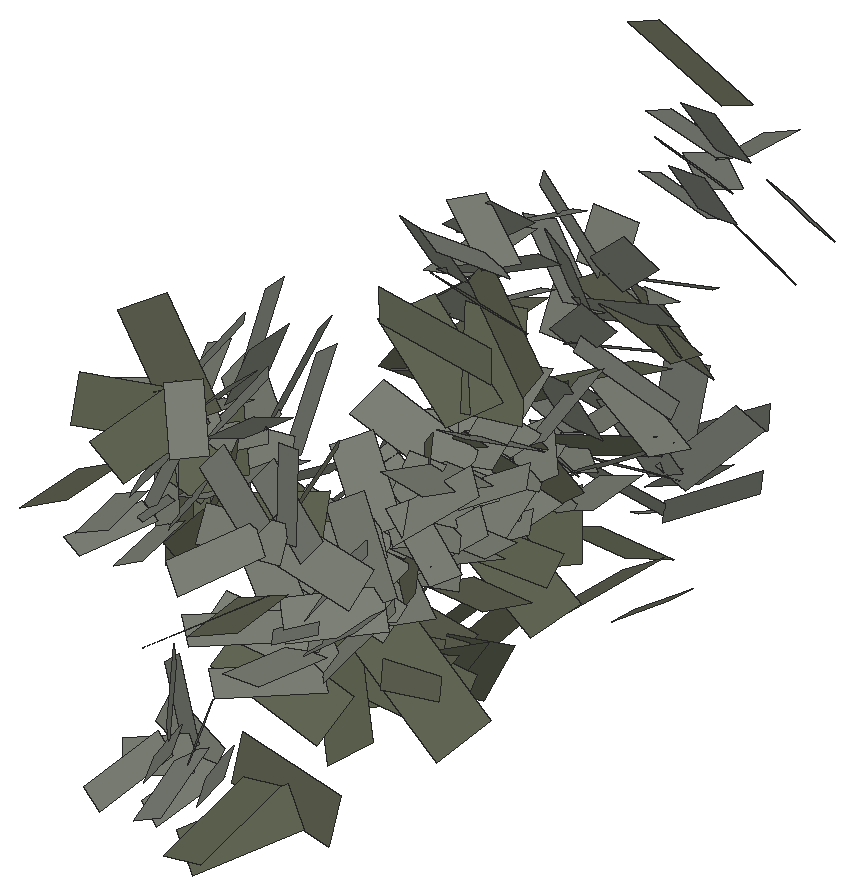
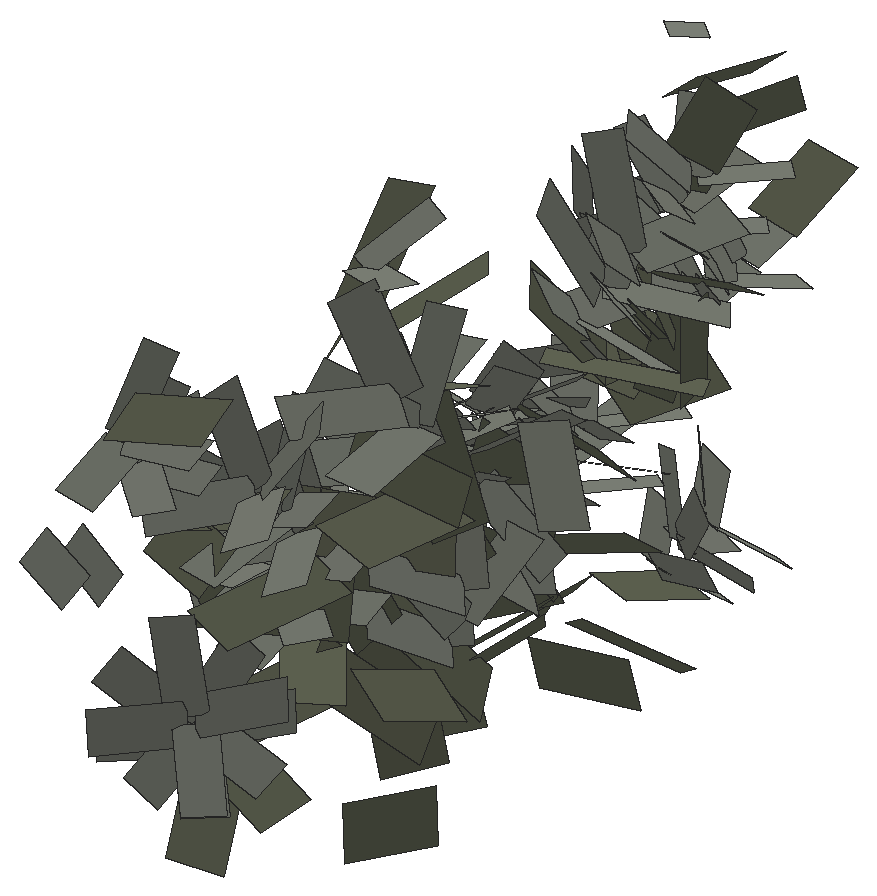
# SketchUp Ruby script. Lengths in inches.
U = 1.inch
M = Sketchup.active_model
def pt(a) = Geom::Point3d.new(a.map { |v| v * U })
def face(e, loops, mat)
  f = e.add_face(loops[0].map { |a| pt(a) })
  loops[1..].each { |l| e.add_face(l.map { |a| pt(a) }).erase! }
  f.material = f.back_material = mat if mat
  f
end
# faces: each face lists its corners as indices into pts; further lists are holes
def faces(e, pts, list, mat = nil) = list.each { |f| face(e, (f[0].is_a?(Array) ? f : [f]).map { |l| l.map { |i| pts[i] } }, mat) }
# xy, xz, yz: faces in a plane at the given z, y or x. An outline is a flat list of corners, or four numbers for a rectangle; further outlines are holes
def ring(l) = l.size == 4 ? [[l[0], l[1]], [l[2], l[1]], [l[2], l[3]], [l[0], l[3]]] : l.each_slice(2).to_a
def flat(e, list, mat, &to3) = list.each { |f| face(e, (f[0].is_a?(Array) ? f : [f]).map { |l| ring(l).map { |u, v| to3.(u, v) } }, mat) }
def xy(e, z, list, mat = nil) = flat(e, list, mat) { |x, y| [x, y, z] }
def xz(e, y, list, mat = nil) = flat(e, list, mat) { |x, z| [x, y, z] }
def yz(e, x, list, mat = nil) = flat(e, list, mat) { |y, z| [x, y, z] }
def lines(e, pts, list) = list.each { |a, b| e.add_line(pt(pts[a]), pt(pts[b])) }
# prism: a flat outline (further loops are holes) pulled along v
def prism(e, loops, v, mat = nil)
  f = face(e, loops, mat); d = Geom::Vector3d.new(v.map { |x| x * U })
  f.pushpull(f.normal.samedirection?(d) ? d.length : -d.length)
end
def box(e, o, s, mat = nil) = prism(e, [[o, [o[0] + s[0], o[1], o[2]], [o[0] + s[0], o[1] + s[1], o[2]], [o[0], o[1] + s[1], o[2]]]], [0, 0, s[2]], mat)
def at(x, y, z, deg = 0) = Geom::Transformation.translation(pt([x, y, z])) * Geom::Transformation.rotation(ORIGIN, Z_AXIS, deg.degrees)
def axes(o, x, y, z) = Geom::Transformation.new([*x, 0, *y, 0, *z, 0, *pt(o).to_a, 1])
def part(name) = M.definitions.add(name)
# library, detail: a bought-in or finely detailed component or shape, given as its bounding box
def library(name, o, s) = part(name).tap { |d| box(d.entities, o, s) }
def detail(e, o, s) = box(e.add_group.entities, o, s)
def put(e, d, t, mat = nil) = e.add_instance(d, t).tap { |i| i.material = mat if mat }
def group(e, t, mat = nil) = e.add_group.tap { |g| g.transformation = t; g.material = mat if mat }.entities
root = M.entities
M.materials.add("viburnumblaasdfas0df1w06d").color = [98, 102, 84]
M.materials.add("viburnumbladsadfasdfad0w122").color = [125, 129, 119]
c1 = part("Component\#315")
p = [[0.25,0,0],[2.05,0.01,0.35],[1.81,4.2,1.66],[0,4.19,1.3125]]
faces(c1.entities,p,[[0,1,2,3]],"viburnumbladsadfasdfad0w122")
c2 = part("viburnumblad2")
put(c2.entities,c1,axes([-19.23,-4.49,-32.18],[83.35428,0,0],[0,79.38502,0],[0,0,83.35428]))
c3 = part("Component\#314")
p = [[0.14,0,0],[2.58,0.05,0.25],[2.44,5.11,2.64],[0,5.05,2.39]]
faces(c3.entities,p,[[0,1,2,3]],"viburnumblaasdfas0df1w06d")
c4 = part("viburnumblad1\#2")
put(c4.entities,c3,axes([-37.25,6.23,19.31],[75.98784,0,0],[0,65.50676,0],[0,0,75.98784]))
put(root,c2,axes([1222.73,192.29,27.47],[-0.00725,0.00846,-0.00094],[-0.008,-0.0072,-0.00303],[-0.00289,-0.00129,0.01072]))
put(root,c2,axes([1222.07,209.96,14.87],[-0.01264,0.00008,-0.0032],[-0.00094,-0.01268,0.00342],[-0.00306,0.00351,0.01217]))
put(root,c4,axes([1221.25,195.38,17.83],[0.00244,-0.01122,0.00057],[0.00459,0.00184,0.0121],[-0.01018,-0.00173,0.00319]))
put(root,c4,axes([1219.0625,212.44,20.56],[0.00379,-0.01036,0.00596],[0.01309,0.006,0.00209],[-0.00395,0.00482,0.01088]))
put(root,c4,axes([1223.68,193.51,22.01],[0.00232,0.01057,0.00577],[-0.01348,0.00407,-0.00203],[-0.00316,-0.00514,0.01068]))
put(root,c2,axes([1222.58,191.05,22.06],[-0.00892,0.00552,-0.00065],[-0.0045,-0.00791,-0.00542],[-0.00314,-0.00411,0.00807]))
put(root,c4,axes([1221.51,190.37,24.46],[-0.01085,-0.00246,-0.00558],[0.00478,-0.01321,-0.00344],[-0.00438,-0.00417,0.00964]))
put(root,c2,axes([1220.42,212.25,24.42],[0.01458,0.00076,-0.00047],[-0.00114,0.0144,-0.00508],[0.00059,0.00521,0.01318]))
put(root,c2,axes([1220.1875,205.77,17.29],[-0.00718,-0.01175,-0.00394],[0.01087,-0.00815,0.00451],[-0.0058,-0.00063,0.01231]))
put(root,c2,axes([1221.58,192.14,20.78],[0.0088,0.00119,0.00472],[-0.00418,0.00904,0.00526],[-0.00322,-0.0061,0.00681]))
put(root,c4,axes([1220.3,210.22,19.54],[0.01555,-0.00131,0.00405],[0.00291,0.01735,-0.00577],[-0.00307,0.00585,0.01401]))
put(root,c2,axes([1219.83,206.21,13.64],[0.012,-0.00837,0.00311],[0.00592,0.01032,0.00492],[-0.00527,-0.00304,0.01219]))
put(root,c2,axes([1222.95,191.44,10.55],[-0.00876,0.00688,0.00103],[-0.00474,-0.00469,-0.00897],[-0.00509,-0.00746,0.00659]))
put(root,c2,axes([1223.27,192.46,9.38],[-0.0033,0.00751,0.0076],[-0.0089,0.00112,-0.00498],[-0.00448,-0.00819,0.00616]))
put(root,c2,axes([1223.96,196.57,24.04],[-0.00774,0.01238,-0.00167],[-0.01057,-0.00772,-0.00819],[-0.0074,-0.00296,0.01235]))
put(root,c2,axes([1219.69,206.34,15.31],[0.00305,-0.01398,-0.00068],[0.01153,0.00223,0.00588],[-0.00601,-0.00193,0.01207]))
put(root,c2,axes([1222.5625,196.9,23.07],[0.00909,0.00693,0.00924],[-0.00802,0.01085,-0.00026],[-0.00757,-0.00532,0.01142]))
put(root,c2,axes([1219.79,211.27,15.82],[0.00854,-0.00917,0.00359],[0.00887,0.00923,0.00245],[-0.00426,0.00084,0.01229]))
put(root,c2,axes([1222.37,193.4,24.57],[0.00793,0.00729,0.0045],[-0.0069,0.00732,0.00029],[-0.00293,-0.00317,0.01031]))
put(root,c2,axes([1221.25,197.5625,24.79],[0.0119,-0.00385,0.00772],[-0.0001,0.01309,0.00669],[-0.00863,-0.00547,0.01057]))
put(root,c2,axes([1223.11,193.72,8.56],[0.00419,0.0043,0.00836],[-0.00938,0.00585,0.00169],[-0.00405,-0.0083,0.0063]))
put(root,c2,axes([1223.71,193.16,24.98],[-0.00696,0.00812,-0.0009],[-0.00864,-0.00777,-0.00327],[-0.00289,-0.00129,0.01072]))
put(root,c4,axes([1221.13,209.875,9.59],[0.01227,-0.00323,0.0066],[0.00379,0.01612,0.00085],[-0.00658,0.00088,0.01266]))
put(root,c2,axes([1222.02,193.4,9.54],[0.00908,-0.00221,0.00614],[-0.004,0.00655,0.00828],[-0.00518,-0.00884,0.00448]))
put(root,c2,axes([1222.11,191,23.36],[-0.00916,-0.00124,-0.00492],[0.00298,-0.00959,-0.00307],[-0.00406,-0.0039,0.00779]))
put(root,c2,axes([1221.35,210.98,16.26],[-0.00933,-0.00906,-0.00093],[0.0081,-0.00886,0.00508],[-0.00417,0.00306,0.01196]))
put(root,c2,axes([1223.32,196.47,25.98],[-0.0119,0.00385,-0.00772],[-0.00199,-0.01402,-0.00394],[-0.0084,-0.00214,0.01187]))
put(root,c2,axes([1223.97,197.06,21.96],[0.00099,0.01426,0.00559],[-0.01157,0.00302,-0.00566],[-0.00706,-0.00428,0.01216]))
put(root,c4,axes([1220.76,211.57,18.54],[-0.00969,-0.0086,0.00402],[0.01095,-0.00941,0.00625],[-0.00101,0.00665,0.01178]))
put(root,c4,axes([1221.8,210.67,4.14],[0.00403,-0.00389,0.01235],[0.00756,0.01368,0.00184],[-0.01119,0.00546,0.00538]))
put(root,c2,axes([1221.06,192.11,22],[0.00892,-0.00552,0.00065],[0.00374,0.00694,0.00752],[-0.00413,-0.00589,0.00653]))
put(root,c2,axes([1223,212.26,24.42],[-0.01458,-0.00076,0.00047],[0.00121,-0.01217,0.00796],[0.00032,0.00837,0.01162]))
put(root,c4,axes([1222.82,192.68,25.68],[0.01074,0.00549,0.00552],[-0.0086,0.00502,0.01173],[0.00238,-0.01127,0.00657]))
put(root,c2,axes([1221.75,193.53,25.78],[0.0105,-0.00104,0.00371],[-0.00021,0.00971,0.00332],[-0.00385,-0.00347,0.00991]))
put(root,c4,axes([1223.4375,194.61,20.03],[0.00961,0.00314,0.00694],[-0.00599,0.01265,0.00258],[-0.0056,-0.00466,0.00986]))
put(root,c2,axes([1221.25,206.29,14.25],[-0.00599,-0.01069,-0.00483],[0.01087,-0.00815,0.00451],[-0.00654,-0.00189,0.01181]))
put(root,c2,axes([1221.54,192.76,11.03],[0.00876,-0.00688,-0.00103],[0.00337,0.00275,0.0103],[-0.00608,-0.00838,0.00422]))
put(root,c2,axes([1220.88,211.25,14.33],[-0.00055,-0.01289,0.00188],[0.01116,0.00015,0.00431],[-0.00466,0.00195,0.01201]))
put(root,c2,axes([1221.09,191.84,23.41],[0.00345,-0.00905,-0.004],[0.00865,0.00062,0.00578],[-0.00475,-0.00515,0.0067]))
put(root,c2,axes([1220.82,210.8,12.8],[0.00892,-0.00957,0.00375],[0.00799,0.0083,0.0022],[-0.00426,0.00084,0.01229]))
put(root,c2,axes([1223.58,193.3,26.46],[-0.0105,0.00104,-0.00371],[-0.00071,-0.0111,-0.00111],[-0.00379,-0.00081,0.01049]))
put(root,c2,axes([1224.17,193.45,9.07],[-0.00914,0.00718,0.00108],[-0.00427,-0.00422,-0.00808],[-0.00509,-0.00746,0.00659]))
put(root,c2,axes([1224.48,216.68,22.27],[0.00139,0.01031,-0.00841],[-0.01248,0.00393,0.00276],[0.0046,0.00756,0.01003]))
put(root,c2,axes([1222.14,210.64,13.26],[-0.00812,-0.00859,-0.00204],[0.0081,-0.00886,0.00508],[-0.00515,0.00206,0.01179]))
put(root,c2,axes([1223.05,192.26,21.66],[-0.00798,-0.00075,-0.00527],[0.00298,-0.00959,-0.00307],[-0.00502,-0.00401,0.00721]))
put(root,c2,axes([1222.11,192.34,22.6],[-0.00404,-0.00727,-0.00631],[0.00772,-0.00559,0.00142],[-0.00472,-0.00433,0.00722]))
put(root,c4,axes([1226.73,197.8,19.48],[-0.0074,0.01393,0.00333],[-0.01491,-0.00558,-0.00981],[-0.00631,-0.00654,0.01332]))
put(root,c2,axes([1220.74,214.07,25.5625],[0.01112,-0.00864,0.0042],[0.00948,0.01048,-0.0033],[-0.0007,0.0056,0.01299]))
put(root,c4,axes([1224.71,190.98,26.64],[-0.0017,0.006,0.01056],[-0.01273,-0.00619,0.00147],[0.00521,-0.00927,0.00611]))
put(root,c2,axes([1220.92,212.42,22.46],[0.01161,-0.00902,0.00438],[0.00853,0.00943,-0.00297],[-0.0007,0.0056,0.01299]))
put(root,c2,axes([1223.64,216.14,20.79],[0.00973,0.00497,-0.00674],[-0.00836,0.01112,-0.00387],[0.00402,0.00678,0.0108]))
put(root,c4,axes([1223.28,195.82,17.98],[-0.00329,-0.00864,-0.00687],[0.00632,-0.00867,0.00771],[-0.00921,-0.00096,0.00528]))
put(root,c2,axes([1221.68,193.99,27.4375],[0.00725,-0.00846,0.00094],[0.00707,0.00667,0.00553],[-0.00474,-0.00299,0.00967]))
put(root,c2,axes([1223.66,192.95,10.53],[-0.00908,0.00221,-0.00614],[0.00272,-0.00885,-0.00722],[-0.00599,-0.007,0.00633]))
put(root,c2,axes([1222.98,193.62,27.85],[-0.00759,-0.00699,-0.00431],[0.00673,-0.00866,0.00218],[-0.0047,-0.00111,0.01008]))
put(root,c4,axes([1225.1875,207.38,7.73],[-0.00681,0.00895,0.00759],[-0.01184,-0.01026,0.00148],[0.00579,-0.00507,0.01117]))
put(root,c4,axes([1222.63,194.22,19.52],[0.00733,-0.00886,0.00054],[0.00689,0.00642,0.00923],[-0.00652,-0.00466,0.00706]))
put(root,c2,axes([1222.17,192.99,21.61],[0.0036,-0.00945,-0.00418],[0.00778,0.00056,0.0052],[-0.00475,-0.00515,0.0067]))
put(root,c4,axes([1221.83,207.72,8.33],[0.00765,-0.01303,0.00422],[0.01267,0.01016,0.00822],[-0.00817,-0.00039,0.01254]))
put(root,c2,axes([1222.74,192.33,11.63],[-0.00409,-0.00375,-0.00971],[0.008,-0.0078,-0.00036],[-0.00665,-0.00708,0.00553]))
put(root,c4,axes([1226.97,198.58,16.59],[0.00378,0.01126,0.01091],[-0.0152,0.00977,-0.00482],[-0.0086,-0.00789,0.01113]))
put(root,c2,axes([1224,218.24,23.4],[0.01014,0.00518,-0.00703],[-0.00774,0.0103,-0.00358],[0.00402,0.00678,0.0108]))
put(root,c2,axes([1221.43,213.46,23.79],[0.00115,-0.01298,0.0064],[0.01333,0.00146,0.00097],[-0.00132,0.00669,0.01246]))
put(root,c2,axes([1225.58,217.65,23.39],[-0.00818,0.0094,-0.00487],[-0.00969,-0.00417,0.00823],[0.00426,0.00856,0.00935]))
put(root,c2,axes([1222.49,212.38,22.59],[-0.0086,-0.00967,0.00326],[0.01109,-0.00774,0.00569],[-0.00192,0.00675,0.01234]))
put(root,c2,axes([1225.88,221.5,14.25],[-0.00504,0.005,-0.01036],[-0.01063,-0.00635,0.00211],[-0.0044,0.00962,0.00678]))
put(root,c4,axes([1226.52,198.56,4.4375],[0.00278,0.00293,0.01264],[-0.01346,0.00734,0.00126],[-0.00579,-0.01128,0.00389]))
put(root,c2,axes([1223.2,198.44,21.99],[0.01174,-0.00298,0.00601],[-0.0001,0.01309,0.00669],[-0.00729,-0.00586,0.01134]))
put(root,c2,axes([1222.58,213.89,25.64],[-0.0095,-0.00972,0.00486],[0.01109,-0.00774,0.00569],[-0.0009,0.00784,0.01189]))
put(root,c2,axes([1225.24,197.82,23.11],[-0.01142,0.0037,-0.00741],[-0.00214,-0.01514,-0.00425],[-0.0084,-0.00214,0.01187]))
put(root,c4,axes([1220.96,210.23,16.76],[0.00743,-0.01098,0.00888],[0.01612,0.00899,-0.00172],[-0.00302,0.0089,0.01251]))
put(root,c2,axes([1222.55,198.16,25.98],[-0.00095,-0.01366,-0.00535],[0.01077,-0.00429,0.00904],[-0.00996,-0.00334,0.01028]))
put(root,c4,axes([1226.56,196.49,6.2],[-0.00836,0.0066,0.00609],[-0.00962,-0.00288,-0.01008],[-0.00344,-0.01004,0.00615]))
put(root,c2,axes([1222.5,194.54,24.95],[0.0071,-0.00744,-0.0001],[0.00707,0.00667,0.00553],[-0.00393,-0.00389,0.00972]))
put(root,c2,axes([1224.97,195.69,15.58],[0.00865,0.00796,0.00491],[-0.00918,0.00854,0.00232],[-0.00184,-0.00511,0.01153]))
put(root,c2,axes([1226.24,195.86,14.17],[-0.00016,0.01206,0.00411],[-0.0133,0.00032,-0.00146],[-0.00141,-0.0041,0.01199]))
put(root,c2,axes([1222.7,193.74,10.75],[0.0033,-0.00751,-0.0076],[0.00833,-0.00317,0.00675],[-0.00669,-0.00765,0.00466]))
put(root,c4,axes([1226.85,197.47,9.74],[0.00263,0.01141,0.00764],[-0.01577,0.00377,-0.0002],[-0.00192,-0.0074,0.01171]))
put(root,c4,axes([1227.07,224.13,28.62],[-0.00083,0.01216,-0.00686],[-0.01618,-0.00142,-0.00053],[-0.00101,0.00652,0.01095]))
put(root,c4,axes([1225.52,195.3125,17.19],[-0.00905,0.00252,-0.00817],[0.0005,-0.01365,-0.00475],[-0.00803,-0.00297,0.00749]))
put(root,c2,axes([1222.67,198.8125,23.86],[0.00774,-0.01238,0.00167],[0.00805,0.00648,0.01066],[-0.00962,-0.00465,0.01009]))
put(root,c2,axes([1224.63,221.47,13.27],[0.01002,0.00748,-0.00127],[-0.0057,0.00603,-0.00944],[-0.00501,0.0081,0.0082]))
put(root,c2,axes([1226.03,220.25,13.03],[0.00352,0.00882,-0.00823],[-0.01182,-0.0007,-0.00581],[-0.00432,0.00892,0.00772]))
put(root,c4,axes([1225.64,204.97,8.35],[-0.01009,0.00576,0.00864],[-0.00958,-0.01423,-0.00203],[0.00708,-0.00619,0.01118]))
put(root,c2,axes([1222.81,194.5,26.42],[-0.00024,-0.01092,-0.00238],[0.01005,-0.00131,0.00499],[-0.0051,-0.00202,0.00975]))
put(root,c2,axes([1224.16,198.06,24.74],[-0.00909,-0.00693,-0.00924],[0.00664,-0.01276,0.00304],[-0.00946,-0.0023,0.01102]))
put(root,c2,axes([1225.72,205,16.11],[0.00269,0.01067,0.0031],[-0.01059,0.00139,0.00439],[0.00368,-0.00386,0.01011]))
put(root,c2,axes([1226.52,195.33,15.84],[-0.00888,0.0091,0.0009],[-0.00895,-0.0084,-0.00345],[-0.00187,-0.00303,0.01224]))
put(root,c4,axes([1222.46,210.67,7.43],[0.00413,-0.01232,0.00597],[0.01417,0.00711,0.00487],[-0.00618,0.00389,0.01229]))
put(root,c2,axes([1226.64,213.81,18.03],[-0.00041,0.01136,-0.00703],[-0.01336,-0.0005,-0.00003],[-0.00029,0.00703,0.01137]))
put(root,c2,axes([1226.28,205.55,14.79],[-0.00563,0.00838,0.00295],[-0.00922,-0.00664,0.00128],[0.00288,-0.0019,0.0109]))
put(root,c4,axes([1222.66,215.1875,17.48],[0.01373,-0.0042,0.00303],[0.00601,0.01319,-0.00893],[-0.00014,0.00827,0.01212]))
put(root,c4,axes([1224.22,200.03,12.78],[0.00372,-0.01109,0.0102],[0.00971,0.0119,0.0094],[-0.01253,0.00356,0.00844]))
put(root,c4,axes([1225.8125,195.63,8.18],[-0.01158,0.00263,-0.00305],[0.00041,-0.00999,-0.01013],[-0.00401,-0.00833,0.00806]))
put(root,c2,axes([1223.86,194.4,10.08],[-0.00392,-0.0036,-0.00932],[0.00864,-0.00842,-0.00039],[-0.00665,-0.00708,0.00553]))
put(root,c2,axes([1226.52,200.76,16.53],[-0.00038,0.01114,0.00561],[-0.01176,-0.00241,0.0034],[0.00455,-0.00528,0.01006]))
put(root,c4,axes([1227.16,205.75,21.32],[0.00623,0.01349,0.00121],[-0.0157,0.00724,0.00014],[-0.00044,-0.00098,0.01352]))
put(root,c2,axes([1225.68,196.92,12.76],[0.00904,0.00831,0.00513],[-0.00826,0.00768,0.00209],[-0.00184,-0.00511,0.01153]))
put(root,c2,axes([1223.65,217.77,21.63],[0.01295,-0.00298,-0.00152],[0.00183,0.01176,-0.00745],[0.00286,0.00667,0.01124]))
put(root,c2,axes([1226.75,204.72,17.35],[-0.00577,0.00885,0.00437],[-0.00922,-0.00664,0.00128],[0.00353,-0.00288,0.01049]))
put(root,c2,axes([1225.92,217.15,21.47],[-0.01295,0.00298,0.00152],[-0.00101,-0.00935,0.0097],[0.0032,0.00918,0.00919]))
put(root,c4,axes([1222.73,208.67,14.24],[-0.01012,-0.01025,0.00891],[0.01634,-0.00922,0.0075],[0.00063,0.01164,0.0125]))
put(root,c2,axes([1227.41,212.35,15.09],[-0.00039,0.0109,-0.00675],[-0.01442,-0.00054,-0.00004],[-0.00029,0.00703,0.01137]))
put(root,c2,axes([1227.46,204.78,19.6],[0,0.01516,0.00154],[-0.01516,-0.00015,0.00148],[0.00149,-0.00153,0.01509]))
put(root,c2,axes([1227.26,196.71,13.04],[-0.00853,0.00873,0.00086],[-0.00967,-0.00907,-0.00372],[-0.00187,-0.00303,0.01224]))
put(root,c2,axes([1227.42,219.57,12.26],[-0.00484,0.0048,-0.00995],[-0.01148,-0.00686,0.00228],[-0.0044,0.00962,0.00678]))
put(root,c4,axes([1227.75,216.99,10.14],[0.00536,0.01158,-0.00521],[-0.01304,0.00197,-0.00903],[-0.0059,0.00728,0.01011]))
put(root,c4,axes([1226.25,198.94,7.68],[0.01152,0.00345,0.00714],[-0.0073,0.01349,0.00527],[-0.00481,-0.00695,0.01113]))
put(root,c4,axes([1226.02,190.36,28.4],[-0.00973,0.00003,0.00746],[-0.00524,-0.01136,-0.00678],[0.00594,-0.00739,0.00778]))
put(root,c2,axes([1226.36,213.28,16.27],[0.00906,0.00899,-0.00397],[-0.01029,0.00825,-0.00478],[-0.00073,0.006,0.01192]))
put(root,c2,axes([1227.01,201.79,15.36],[-0.00848,0.00652,0.00394],[-0.00785,-0.00971,-0.00119],[0.00311,-0.00363,0.01115]))
put(root,c2,axes([1225.46,205.18,17.8],[0.00958,0.00624,0.00001],[-0.00544,0.00834,0.00562],[0.00306,-0.00472,0.00995]))
put(root,c2,axes([1227.32,223.23,27.34],[0.00014,0.01001,-0.00619],[-0.01174,-0.00053,-0.00107],[-0.00123,0.00599,0.0089]))
put(root,c4,axes([1226.75,211.05,11.83],[0.01166,0.00889,0.00003],[-0.00952,0.01251,-0.00648],[-0.00341,0.00442,0.01356]))
put(root,c2,axes([1226.12,200.5,18.26],[0.00829,0.0091,0.00248],[-0.00839,0.00593,0.00669],[0.00415,-0.0063,0.00965]))
put(root,c4,axes([1224.15,195.42,18.83],[-0.001,-0.01064,-0.00433],[0.01169,-0.00333,0.00541],[-0.00539,-0.00308,0.00855]))
put(root,c2,axes([1226.91,207.9,28.46],[0.00564,0.00974,-0.00221],[-0.01091,0.00622,-0.00021],[0.00111,0.00263,0.01119]))
put(root,c4,axes([1224.46,196.42,18.27],[0.00803,-0.00983,0.00384],[0.00868,0.0101,0.00771],[-0.00745,-0.00186,0.01082]))
put(root,c2,axes([1227.2,221.0625,13],[-0.01065,-0.00175,-0.00643],[-0.00418,-0.00769,0.00902],[-0.00519,0.00978,0.00593]))
put(root,c2,axes([1227.84,213.33,16.52],[-0.00964,0.00707,-0.00598],[-0.00922,-0.00808,0.00531],[-0.0008,0.00796,0.01071]))
put(root,c2,axes([1225.12,196.86,14.22],[0.0124,-0.0008,0.00284],[-0.00048,0.01054,0.00506],[-0.0029,-0.00547,0.01114]))
put(root,c2,axes([1226.09,219.47,11.375],[0.01046,0.00781,-0.00132],[-0.00513,0.00543,-0.00849],[-0.00501,0.0081,0.0082]))
put(root,c4,axes([1224.7,210.02,5.28],[-0.01097,-0.01069,0.00215],[0.01213,-0.01096,0.00739],[-0.00308,0.00597,0.01392]))
put(root,c2,axes([1226.8,205.43,17.71],[0.01077,0.01069,0.00135],[-0.01074,0.01048,0.00267],[0.00094,-0.00284,0.01494]))
put(root,c4,axes([1225.96,195.64,17.28],[-0.01126,-0.00328,-0.00424],[0.0051,-0.0131,-0.00341],[-0.00278,-0.00386,0.0103]))
put(root,c2,axes([1227.63,200.47,17.88],[-0.00883,0.00666,0.00546],[-0.00785,-0.00971,-0.00119],[0.00409,-0.00438,0.01062]))
put(root,c4,axes([1224.47,208.13,6.3],[-0.00857,-0.01458,-0.00131],[0.01562,-0.00975,0.00697],[-0.00558,0.00226,0.01502]))
put(root,c4,axes([1228.875,203.89,8.22],[0.00192,0.00886,0.01301],[-0.01818,-0.00012,0.00276],[0.00142,-0.01315,0.00875]))
put(root,c2,axes([1226.94,222.63,25.96],[0.00824,0.00797,-0.00286],[-0.00838,0.00693,-0.00484],[-0.00165,0.00508,0.00936]))
put(root,c2,axes([1228.01,221.74,25.32],[0.00025,0.00856,-0.00655],[-0.01174,-0.00053,-0.00107],[-0.00121,0.00703,0.00818]))
put(root,c2,axes([1227.07,205.89,16.08],[-0.01085,0.00184,0.00308],[-0.00218,-0.01013,-0.00164],[0.00269,-0.00234,0.01086]))
put(root,c4,axes([1223.98,212.31,12.6875],[-0.01045,-0.00476,0.01095],[0.01292,-0.01059,0.00773],[0.00429,0.01208,0.00936]))
put(root,c2,axes([1223.96,217.4375,19.74],[0.00854,-0.00981,0.00509],[0.00939,0.0055,-0.00515],[0.00179,0.0073,0.01107]))
put(root,c2,axes([1227.99,208.23,19.69],[0.00259,0.01229,-0.00001],[-0.01185,0.00249,-0.00335],[-0.00327,0.0007,0.01211]))
put(root,c2,axes([1225.35,217.05,19.77],[-0.00947,-0.00564,0.00547],[0.00849,-0.00835,0.00609],[0.00092,0.00846,0.01032]))
put(root,c4,axes([1223.01,214.53,14.85],[0.00481,-0.00968,0.00992],[0.01607,0.00349,-0.00438],[0.00046,0.01061,0.01012]))
put(root,c4,axes([1227.24,206.37,21.54],[0.00918,0.0099,-0.00625],[-0.01245,0.01197,0.0007],[0.0045,0.00408,0.01216]))
put(root,c4,axes([1228.5625,206.42,23.73],[-0.00859,0.01076,0.00042],[-0.01222,-0.00981,0.0027],[0.00229,0.0015,0.01233]))
put(root,c2,axes([1225.36,220.76,11.8125],[0.01065,0.00175,0.00643],[0.00257,0.00902,-0.00671],[-0.00605,0.00763,0.00794]))
put(root,c2,axes([1228.73,205.14,17.72],[-0.01077,0.01075,0.00083],[-0.01084,-0.01091,0.00051],[0.00094,-0.00022,0.01521]))
put(root,c2,axes([1227.29,196.66,14.74],[-0.0124,0.0008,-0.00284],[-0.0002,-0.01247,-0.00265],[-0.00294,-0.00253,0.01214]))
put(root,c2,axes([1225.64,214.88,17.2],[0.01322,0.00136,0.00142],[-0.00064,0.01212,-0.00561],[-0.00186,0.00548,0.01205]))
put(root,c2,axes([1226.55,222.63,13.37],[-0.01002,-0.00748,0.00127],[0.00432,-0.00389,0.01114],[-0.00624,0.00932,0.00567]))
put(root,c2,axes([1225.17,206.24,16.67],[0.01085,-0.00184,-0.00308],[0.00296,0.01015,0.00436],[0.00203,-0.00494,0.01011]))
put(root,c2,axes([1225.56,201.78,17.27],[0.01211,0.00173,-0.00211],[0,0.01038,0.00684],[0.00312,-0.00685,0.00964]))
put(root,c2,axes([1227.48,190.83,22.61],[0.00766,0.00322,0.00823],[-0.00853,0.00606,0.00527],[-0.00262,-0.00929,0.00521]))
put(root,c2,axes([1228.25,208.09,28.43],[-0.01136,0.00626,-0.00167],[-0.00565,-0.00941,0.00229],[-0.00013,0.00352,0.01104]))
put(root,c4,axes([1226.22,207.9375,10.25],[-0.01133,-0.00353,0.00405],[0.00312,-0.01382,-0.0033],[0.00465,-0.0017,0.01152]))
put(root,c2,axes([1228.58,196.44,17.38],[0.00252,0.00942,0.00914],[-0.01307,0.00092,0.00265],[0.00124,-0.00944,0.00938]))
put(root,c2,axes([1224.76,218.45,20.75],[-0.00139,-0.01031,0.00841],[0.01214,-0.00182,-0.00024],[0.00145,0.00829,0.0104]))
put(root,c2,axes([1228.57,222.79,26.24],[-0.00804,0.00619,-0.0059],[-0.0078,-0.0066,0.00358],[-0.00163,0.0068,0.00829]))
put(root,c2,axes([1224.45,219.46,22.32],[0.00818,-0.0094,0.00487],[0.01043,0.00611,-0.00572],[0.00179,0.0073,0.01107]))
put(root,c2,axes([1228.74,191.46,21.75],[-0.00034,0.00733,0.00907],[-0.01154,0.00172,-0.00184],[-0.00225,-0.00876,0.00608]))
put(root,c4,axes([1229.78,217.34,20.15],[-0.00128,0.01292,-0.00526],[-0.01614,-0.0018,-0.00049],[-0.00098,0.00473,0.0118]))
put(root,c2,axes([1228.71,198.56,14.99],[0.00219,0.00955,0.00743],[-0.01307,0.00092,0.00265],[0.0015,-0.00837,0.01031]))
put(root,c2,axes([1226.03,218.87,22.3125],[-0.01014,-0.00518,0.00703],[0.00849,-0.00835,0.00609],[0.00203,0.00907,0.00962]))
put(root,c4,axes([1227.9375,201.06,14.21],[0.01183,-0.00442,0.01203],[-0.00182,0.01827,0.0085],[-0.01272,-0.00605,0.01028]))
put(root,c2,axes([1225.3,222.6,12.39],[0.00504,-0.005,0.01036],[0.00925,0.00849,-0.00041],[-0.00684,0.0078,0.00709]))
put(root,c2,axes([1228.88,190.32,22.73],[-0.00814,0.00715,0.0046],[-0.00805,-0.00423,-0.00746],[-0.00268,-0.00803,0.00677]))
put(root,c2,axes([1226.69,206.7,15],[-0.01,-0.00652,-0.00001],[0.00542,-0.00831,-0.00274],[0.00166,-0.00256,0.01102]))
put(root,c2,axes([1225.22,197.17,16.15],[0.00888,-0.0091,-0.0009],[0.00823,0.00741,0.00631],[-0.00398,-0.00497,0.01104]))
put(root,c2,axes([1226.28,213.36,14.33],[0.0138,0.00142,0.00148],[-0.00058,0.0109,-0.00504],[-0.00186,0.00548,0.01205]))
put(root,c2,axes([1227.98,214.78,17.66],[-0.01322,-0.00136,-0.00142],[0.00017,-0.01043,0.00835],[-0.00196,0.00824,0.01034]))
put(root,c4,axes([1229.54,217.91,20.07],[0.00337,0.00858,-0.01052],[-0.01574,0.00327,-0.00237],[0.0008,0.00999,0.00793]))
put(root,c2,axes([1227.6875,202.0625,16.84],[-0.01211,-0.00173,0.00211],[0.00069,-0.01077,-0.00395],[0.00303,-0.00413,0.011]))
put(root,c2,axes([1226.49,224.17,26.55],[0.01151,0.00126,0.00215],[-0.00018,0.01065,-0.00509],[-0.00265,0.00461,0.00939]))
put(root,c2,axes([1229.44,208.35,18.52],[-0.0062,0.01038,-0.0034],[-0.01088,-0.00717,-0.00204],[-0.00346,0.00185,0.01194]))
put(root,c4,axes([1227.99,215.82,7.87],[0.01075,0.00741,0.00439],[-0.00265,0.0107,-0.01157],[-0.00831,0.00706,0.00843]))
put(root,c2,axes([1226.67,189.16,31.06],[-0.00866,-0.00577,-0.00263],[0.00674,-0.00675,-0.0074],[0.00215,-0.00706,0.0084]))
put(root,c2,axes([1226.35,206.35,19.74],[0.01523,-0.00004,0.00037],[-0.00005,0.01486,0.00338],[-0.00037,-0.00338,0.01485]))
put(root,c2,axes([1229.01,208.18,16.75],[0.0027,0.01283,-0.00001],[-0.01066,0.00224,-0.00301],[-0.00327,0.0007,0.01211]))
put(root,c2,axes([1227.87,197.96,16.45],[0.01106,0.0052,0.00541],[-0.00756,0.007,0.00872],[0.00055,-0.01018,0.00865]))
put(root,c2,axes([1226.76,196.81,16.42],[-0.00865,-0.00796,-0.00491],[0.00846,-0.00952,0.00054],[-0.00401,-0.0029,0.01175]))
put(root,c2,axes([1225.34,207.06,15.39],[0.00554,-0.00849,-0.00419],[0.01058,0.00621,0.0014],[0.00119,-0.0044,0.01049]))
put(root,c2,axes([1228.51,224.09,27.11],[-0.01151,-0.00126,-0.00215],[-0.00046,-0.00922,0.00721],[-0.00262,0.00705,0.00788]))
put(root,c2,axes([1225.8,198.17,13.33],[0.00852,-0.00783,-0.00192],[0.00823,0.00741,0.00631],[-0.003,-0.00593,0.01088]))
put(root,c2,axes([1228.09,208.52,17.9375],[0.00987,0.007,0.00339],[-0.00618,0.00957,-0.0018],[-0.0039,-0.00027,0.01194]))
put(root,c4,axes([1230.76,207.78,14.06],[-0.00473,0.01294,-0.00003],[-0.01473,-0.00539,-0.00308],[-0.0025,-0.00088,0.01352]))
put(root,c2,axes([1229.72,197.6875,16.21],[-0.00749,0.00812,0.00752],[-0.01012,-0.00577,-0.00385],[0.00099,-0.00855,0.01022]))
put(root,c2,axes([1228.74,192.86,21.22],[0.00736,0.00309,0.0079],[-0.00921,0.00654,0.0057],[-0.00262,-0.00929,0.00521]))
put(root,c4,axes([1226.46,205.26,11.18],[-0.0111,-0.00766,0.00199],[0.00742,-0.01279,-0.00569],[0.00489,-0.00308,0.01206]))
put(root,c2,axes([1225.56,202.96,16.14],[0.00848,-0.00639,-0.00524],[0.0093,0.00903,0.00402],[0.00207,-0.0066,0.01002]))
put(root,c2,axes([1226.76,206.39,15.91],[0.01462,-0.00004,0.00036],[-0.00005,0.01605,0.00365],[-0.00037,-0.00338,0.01485]))
put(root,c2,axes([1227.32,206.01,17.67],[-0.00958,-0.00624,-0.00001],[0.00602,-0.00923,-0.00305],[0.00166,-0.00256,0.01102]))
put(root,c4,axes([1226.76,210.99,9.1],[0.01294,-0.00163,0.0067],[0.00488,0.01526,-0.00571],[-0.00546,0.00626,0.01208]))
put(root,c2,axes([1229.34,227.08,23.25],[0.00367,0.00526,-0.00978],[-0.01118,0.00267,-0.00269],[0.001,0.0097,0.00482]))
put(root,c4,axes([1230.34,207.59,11.54],[0.00606,0.01155,0.00446],[-0.01316,0.00831,-0.00362],[-0.00493,-0.00229,0.01266]))
put(root,c2,axes([1226.75,221.84,11.66],[-0.00352,-0.00882,0.00823],[0.00998,0.00284,0.00731],[-0.00692,0.00849,0.00615]))
put(root,c2,axes([1229.46,224.64,22.29],[0.00325,0.00384,-0.00943],[-0.01118,0.00267,-0.00269],[0.00139,0.01021,0.00373]))
put(root,c2,axes([1229.35,208.88,20.19],[-0.01136,0.00239,-0.0048],[-0.00314,-0.01208,0.00143],[-0.00434,0.00249,0.01152]))
put(root,c2,axes([1227.1,203.04,15.85],[-0.00866,-0.0095,-0.00259],[0.00823,-0.00655,-0.00374],[0.002,-0.00468,0.01099]))
put(root,c2,axes([1229.92,215.45,17.3],[0.0037,0.01302,-0.00469],[-0.01381,0.00379,-0.00038],[0.0009,0.00462,0.01353]))
put(root,c4,axes([1229.57,207.3,22.99],[-0.00512,0.01258,-0.00225],[-0.01225,-0.00318,0.00944],[0.00707,0.00483,0.00942]))
put(root,c2,axes([1229.03,205.88,19.75],[-0.01523,0.00004,-0.00037],[-0.00005,-0.01523,0.00032],[-0.00037,0.00032,0.01523]))
put(root,c4,axes([1225.83,208.08,12.55],[-0.00529,-0.01137,-0.00003],[0.01295,-0.00601,-0.0028],[0.00218,-0.00104,0.01231]))
put(root,c2,axes([1226.1875,214.59,15.41],[0.00964,-0.00707,0.00598],[0.00804,0.00897,-0.00235],[-0.00301,0.00576,0.01168]))
put(root,c2,axes([1226.03,206.47,18.125],[0.00577,-0.00885,-0.00437],[0.0098,0.00575,0.0013],[0.00119,-0.0044,0.01049]))
put(root,c2,axes([1226.3,206.86,16.6],[-0.00269,-0.01067,-0.0031],[0.01162,-0.00239,-0.00186],[0.00104,-0.00341,0.01086]))
put(root,c2,axes([1229.02,222.47,25.03],[-0.01201,-0.00131,-0.00224],[-0.00042,-0.0083,0.00649],[-0.00262,0.00705,0.00788]))
put(root,c4,axes([1230.4,201.15,8.43],[0.00636,0.01278,0.00656],[-0.01653,0.00548,0.00535],[0.00178,-0.00782,0.01351]))
put(root,c2,axes([1226.33,197.97,14.94],[0.00016,-0.01206,-0.00411],[0.01207,-0.0013,0.00429],[-0.00443,-0.00391,0.01129]))
put(root,c2,axes([1230.6,216.07,19.05],[-0.00715,0.01146,-0.00475],[-0.01239,-0.00628,0.0035],[0.00072,0.00585,0.01305]))
put(root,c2,axes([1226.56,220.51,10.64],[0.00529,-0.00535,0.00878],[0.00925,0.00849,-0.00041],[-0.00626,0.00721,0.00817]))
put(root,c2,axes([1229.25,206.33,16.14],[-0.01389,0,-0.00185],[-0.00005,-0.01523,0.00032],[-0.00201,0.00032,0.0151]))
put(root,c4,axes([1228.82,208.06,25.53],[-0.01366,0.00026,0.00163],[0.00037,-0.01516,0.00432],[0.00177,0.00434,0.01188]))
put(root,c2,axes([1227.43,209.67,19.34],[0.01136,-0.00239,0.0048],[0.002,0.01232,0.0014],[-0.00498,-0.0005,0.01153]))
put(root,c2,axes([1227.91,192.32,22.33],[0.01118,-0.00278,0.00257],[-0.00082,0.00655,0.0102],[-0.00357,-0.00931,0.00467]))
put(root,c2,axes([1226.33,201.92,18.92],[0.00883,-0.00666,-0.00546],[0.00861,0.00836,0.00373],[0.00207,-0.0066,0.01002]))
put(root,c2,axes([1229.81,200.82,17.24],[0.00207,0.01081,-0.00198],[-0.01024,0.00263,0.00364],[0.00398,0.00114,0.01039]))
